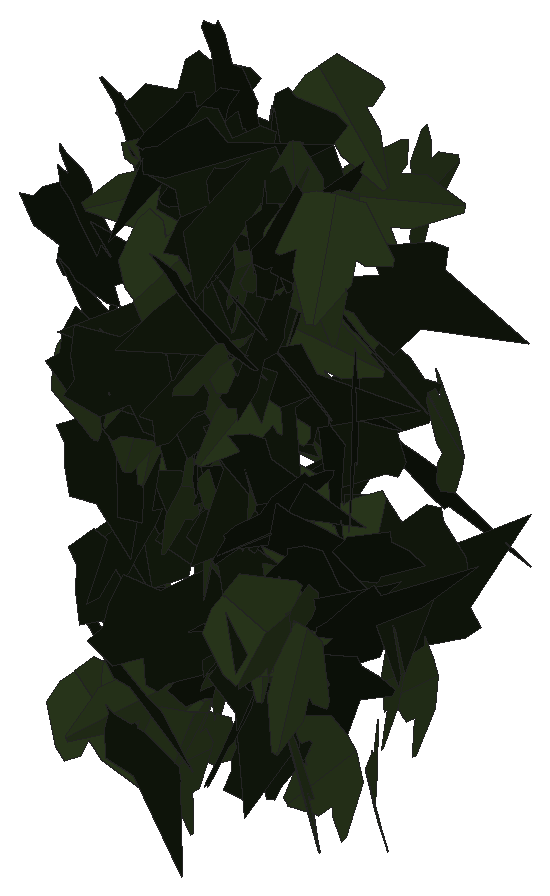
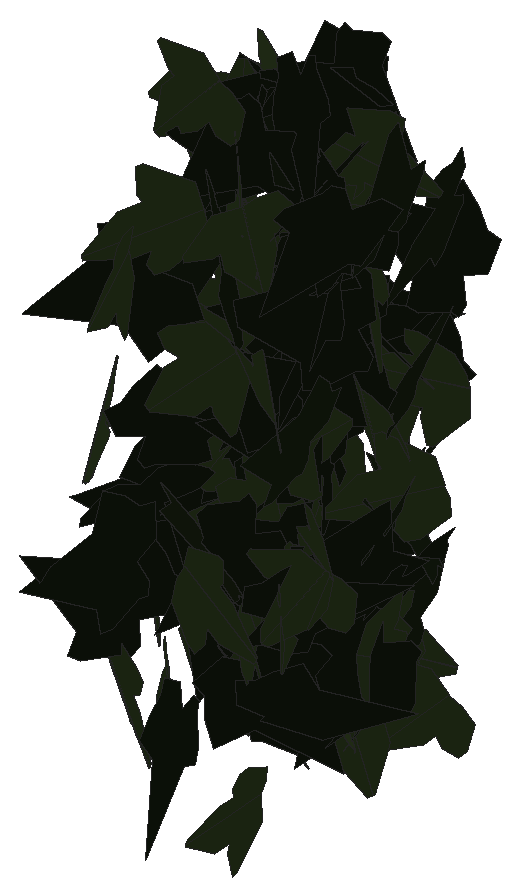
# SketchUp Ruby script. Lengths in inches.
U = 1.inch
M = Sketchup.active_model
def pt(a) = Geom::Point3d.new(a.map { |v| v * U })
def face(e, loops, mat)
  f = e.add_face(loops[0].map { |a| pt(a) })
  loops[1..].each { |l| e.add_face(l.map { |a| pt(a) }).erase! }
  f.material = f.back_material = mat if mat
  f
end
# faces: each face lists its corners as indices into pts; further lists are holes
def faces(e, pts, list, mat = nil) = list.each { |f| face(e, (f[0].is_a?(Array) ? f : [f]).map { |l| l.map { |i| pts[i] } }, mat) }
# xy, xz, yz: faces in a plane at the given z, y or x. An outline is a flat list of corners, or four numbers for a rectangle; further outlines are holes
def ring(l) = l.size == 4 ? [[l[0], l[1]], [l[2], l[1]], [l[2], l[3]], [l[0], l[3]]] : l.each_slice(2).to_a
def flat(e, list, mat, &to3) = list.each { |f| face(e, (f[0].is_a?(Array) ? f : [f]).map { |l| ring(l).map { |u, v| to3.(u, v) } }, mat) }
def xy(e, z, list, mat = nil) = flat(e, list, mat) { |x, y| [x, y, z] }
def xz(e, y, list, mat = nil) = flat(e, list, mat) { |x, z| [x, y, z] }
def yz(e, x, list, mat = nil) = flat(e, list, mat) { |y, z| [x, y, z] }
def lines(e, pts, list) = list.each { |a, b| e.add_line(pt(pts[a]), pt(pts[b])) }
# prism: a flat outline (further loops are holes) pulled along v
def prism(e, loops, v, mat = nil)
  f = face(e, loops, mat); d = Geom::Vector3d.new(v.map { |x| x * U })
  f.pushpull(f.normal.samedirection?(d) ? d.length : -d.length)
end
def box(e, o, s, mat = nil) = prism(e, [[o, [o[0] + s[0], o[1], o[2]], [o[0] + s[0], o[1] + s[1], o[2]], [o[0], o[1] + s[1], o[2]]]], [0, 0, s[2]], mat)
def at(x, y, z, deg = 0) = Geom::Transformation.translation(pt([x, y, z])) * Geom::Transformation.rotation(ORIGIN, Z_AXIS, deg.degrees)
def axes(o, x, y, z) = Geom::Transformation.new([*x, 0, *y, 0, *z, 0, *pt(o).to_a, 1])
def part(name) = M.definitions.add(name)
# library, detail: a bought-in or finely detailed component or shape, given as its bounding box
def library(name, o, s) = part(name).tap { |d| box(d.entities, o, s) }
def detail(e, o, s) = box(e.add_group.entities, o, s)
def put(e, d, t, mat = nil) = e.add_instance(d, t).tap { |i| i.material = mat if mat }
def group(e, t, mat = nil) = e.add_group.tap { |g| g.transformation = t; g.material = mat if mat }.entities
root = M.entities
M.materials.add("efeu1").color = [18, 25, 13]
M.materials.add("efeu2").color = [43, 57, 29]
c1 = part("ivyleaf_9")
p = [[1.54,2.16,1.25],[1.36,2.04,1.19],[-0.21,0.99,0.68],[-0.71,1.11,0.82],[-0.85,0.86,0.67],[-0.8,0.17,0.21],
  [-0.9,-0.01,0.1],[-0.67,-0.16,-0.02],[-0.08,-0.08,-0.05],[-0.03,-0.6,-0.4],[0.65,-0.88,-0.66],[0.83,-0.6,-0.49],
  [1.29,-0.42,-0.43],[1.8125,-0.07,-0.26],[1.21,0.44,0.15]]
faces(c1.entities,p,[[0,1,2,3,4,5,6,7,8,9,10,11,12,13,14]],"efeu1")
c2 = part("ivyleaf_10")
p = [[0,0.5,-0.03],[-0.0625,2.02,-0.43],[-0.19,2.01,-0.46],[-0.54,1.05,-0.29],[-0.52,0.625,-0.18],[-0.83,0.76,-0.28],
  [-1.16,0.64,-0.33],[-1.15,0.33,-0.24],[-0.77,-0.39,0.02],[-0.3,-0.51,0.16],[0.04,-0.48,0.23],[-0.02,2.01,-0.4375],
  [-0.06,2.01,-0.43],[0.04,-0.49,0.23],[0.67,-0.49,0.14],[1.38,0.36,-0.2],[1.375,0.51,-0.24],[0.81,0.65,-0.19],
  [0.62,0.59,-0.15],[0.6,1.09,-0.28],[0.5,1.23,-0.31]]
faces(c2.entities,p,[[0,1,2,3,4,5,6,7,8,9,10],[11,12,0,13,14,15,16,17,18,19,20]],"efeu2")
put(root,c1,axes([28.6875,223.91,213.04],[0.40877,-0.21276,-0.19401],[-0.17176,0.09021,-0.46083],[0.2311,0.44339,0.00067]))
put(root,c1,axes([28.94,224.4375,210.86],[0.14407,-0.45026,0.16281],[-0.02186,0.16366,0.47195],[-0.47829,-0.14311,0.02747]))
put(root,c2,axes([28.55,224.56,210.09],[0.11847,0.08591,0.47811],[0.33881,0.33804,-0.1447],[-0.3481,0.35826,0.02188]))
put(root,c2,axes([28.97,226.4375,211.65],[0.40883,-0.22984,0.17329],[-0.15126,0.08456,0.46901],[-0.2449,-0.43592,-0.00038]))
put(root,c1,axes([28.55,223.95,212.3],[0.14856,-0.10104,0.46661],[0.392,-0.25313,-0.17962],[0.27252,0.41919,0.004]))
put(root,c1,axes([28.66,226.22,211.32],[0.30316,-0.37641,0.12809],[0.08821,-0.09339,-0.48321],[0.3877,0.31558,0.00978]))
put(root,c1,axes([28.73,224.88,213.16],[0.3783,-0.19985,-0.25874],[0.22756,-0.12317,0.42784],[-0.23474,-0.44146,-0.00224]))
put(root,c2,axes([28.67,224.14,207.4375],[0.33561,0.08296,0.36123],[0.34168,0.11955,-0.34491],[-0.14359,0.47836,0.02355]))
put(root,c2,axes([28.94,224.81,208.15],[0.07535,-0.22845,0.43833],[0.17161,-0.40372,-0.23991],[0.46354,0.1866,0.01757]))
put(root,c1,axes([28.87,225.29,213.42],[-0.00267,-0.238,-0.43971],[0.03683,0.43843,-0.23753],[0.49863,-0.03366,0.01519]))
put(root,c2,axes([28.78,225.85,209.67],[-0.0462,0.07315,-0.49246],[0.30942,-0.38324,-0.08596],[-0.39003,-0.3127,-0.00985]))
put(root,c1,axes([29.32,225.95,208.99],[-0.21599,-0.12914,0.43205],[-0.37674,-0.21159,-0.25159],[0.24781,-0.43423,-0.0059]))
put(root,c1,axes([28.89,224.73,209.64],[-0.05666,-0.22028,0.44527],[0.06937,-0.44727,-0.21245],[0.49191,0.03771,0.08125]))
put(root,c1,axes([28.94,224.74,208.25],[0.44801,0.21995,-0.03005],[-0.03031,-0.00644,-0.49904],[-0.21992,0.44898,0.00756]))
put(root,c2,axes([28.69,224,210.99],[-0.07061,-0.0021,-0.49498],[0.48693,-0.09017,-0.06907],[-0.08898,-0.4918,0.01478]))
put(root,c1,axes([28.83,224.09,210.17],[0.25674,-0.42821,-0.0269],[-0.01511,0.0223,-0.49927],[0.42878,0.25718,-0.00149]))
put(root,c1,axes([28.89,224.33,208.97],[0.17941,-0.4226,-0.19804],[-0.06084,0.18918,-0.45881],[0.46272,0.18873,0.01646]))
put(root,c1,axes([29.44,225.82,207.77],[-0.26268,-0.03608,0.42391],[-0.41881,-0.06569,-0.26511],[0.07482,-0.49435,0.00429]))
put(root,c2,axes([28.82,225.89,209.52],[0.36416,0.17833,0.29255],[0.25167,0.15047,-0.40499],[-0.23248,0.44222,0.01983]))
put(root,c1,axes([29.33,224.9,209.03],[-0.41509,-0.26704,0.07993],[0.06882,0.04076,0.49356],[-0.27012,0.42074,0.00292]))
put(root,c1,axes([29.29,223.82,209.22],[-0.34413,0.32724,-0.15648],[-0.12117,0.0996,0.47476],[0.34189,0.36468,0.01075]))
put(root,c2,axes([29.15,224.22,207.93],[0.04653,0.30441,0.39392],[0.07018,0.38767,-0.30787],[-0.49286,0.08394,-0.00665]))
put(root,c2,axes([29.1875,224.55,210.8],[0.45106,-0.20553,0.06559],[0.06059,-0.0252,-0.49567],[0.20706,0.45511,0.00217]))
put(root,c1,axes([29.02,224.04,208.23],[0.37916,-0.32449,0.03065],[0.02319,-0.02004,-0.49906],[0.32511,0.37987,-0.00015]))
put(root,c2,axes([29.51,224.23,207.82],[-0.05387,-0.17407,0.46561],[-0.16039,-0.43721,-0.18201],[0.4705,-0.16897,-0.00874]))
put(root,c2,axes([29.25,225.58,210.72],[-0.00569,-0.05343,0.4971],[0.18139,-0.46349,-0.04774],[0.4659,0.17979,0.02466]))
put(root,c1,axes([29.05,223.89,210.89],[-0.10825,0.03471,0.48691],[0.43525,-0.21892,0.11237],[0.22099,0.44818,0.01718]))
put(root,c2,axes([29.41,225.48,209.28],[0.08997,-0.40958,-0.2723],[-0.02562,0.27254,-0.41841],[0.49117,0.08924,0.02805]))
put(root,c2,axes([29.47,224.28,212.13],[0.30868,-0.25758,-0.29727],[-0.16144,0.26162,-0.39433],[0.35868,0.33943,0.07834]))
put(root,c2,axes([29.5,224.03,211.05],[-0.38838,-0.28696,0.12967],[-0.10056,-0.08209,-0.48285],[0.29841,-0.40114,0.00605]))
put(root,c2,axes([29.74,226.64,209.48],[-0.1779,0.03813,0.46572],[-0.46728,-0.01242,-0.17747],[-0.00196,-0.49839,0.04005]))
put(root,c1,axes([29.63,225.82,208.24],[0.03233,0.22646,-0.4446],[-0.06196,-0.44026,-0.22875],[-0.49509,0.06988,-0.00041]))
put(root,c2,axes([29.6,224.46,207.27],[-0.28853,-0.38483,0.13659],[-0.07791,-0.1123,-0.48096],[0.40085,-0.29883,0.00484]))
put(root,c1,axes([29.62,224.64,209.93],[-0.00253,-0.06778,0.49538],[0.02287,0.49485,0.06782],[-0.49947,0.02301,0.0006]))
put(root,c2,axes([29.46,226.12,206.88],[0.05637,-0.01042,-0.4967],[0.09809,0.49028,0.00084],[0.48703,-0.09753,0.05732]))
put(root,c1,axes([29.82,224.6,211.49],[-0.2655,-0.05561,0.42002],[-0.39578,-0.14438,-0.26929],[0.15123,-0.47546,0.03265]))
put(root,c2,axes([29.84,224.08,213.33],[0.21481,0.03242,-0.45034],[-0.44683,-0.05629,-0.21719],[-0.06478,0.49576,0.00478]))
put(root,c1,axes([29.34,224.15,207.3],[0.19968,-0.45082,0.083],[0.03004,-0.07747,-0.49305],[0.45741,0.20189,-0.00386]))
put(root,c1,axes([30,224.03,211.42],[-0.41401,0.1922,0.2041],[-0.18692,0.08206,-0.45643],[-0.20895,-0.45423,0.0039]))
put(root,c1,axes([29.5,223.78,211.06],[-0.25682,-0.06376,0.42424],[0.42889,-0.02657,0.25564],[-0.01006,0.49521,0.06834]))
put(root,c1,axes([29.29,224.72,211.73],[0.2633,-0.00274,0.42505],[0.41926,0.08394,-0.25918],[-0.06993,0.4929,0.0465]))
put(root,c2,axes([29.74,224.28,210.02],[-0.00079,-0.27761,-0.41585],[-0.00374,0.41584,-0.2776],[0.49999,0.00267,-0.00274]))
put(root,c1,axes([29.5,224.58,210.52],[-0.09786,-0.05019,0.48775],[0.45227,0.18288,0.10956],[-0.1894,0.46264,0.00961]))
put(root,c2,axes([29.74,225.67,208.66],[0.09486,-0.48546,0.07298],[0.01243,-0.07194,-0.49464],[0.49076,0.09566,-0.00158]))
put(root,c1,axes([29.91,224.75,214.32],[0.24472,-0.00269,-0.43601],[-0.43568,-0.02129,-0.2444],[-0.01725,0.49954,-0.01277]))
put(root,c1,axes([29.8,226.81,208.08],[0.35829,-0.03495,-0.347],[-0.34354,0.05031,-0.35979],[0.06006,0.49623,0.01204]))
put(root,c1,axes([29.78,224.66,212.01],[0.39745,0.01618,-0.30294],[-0.30329,0.00961,-0.3974],[-0.00703,0.49965,0.01745]))
put(root,c1,axes([29.41,224.85,213.02],[0.09089,0.00062,-0.49167],[0.48585,0.07658,0.08991],[0.07542,-0.4941,0.01332]))
put(root,c2,axes([29.64,224.42,206.95],[0.14649,-0.26393,-0.3986],[0.25004,-0.31302,0.29916],[-0.40745,-0.28698,0.04028]))
put(root,c1,axes([29.99,224.07,214.15],[-0.16598,0.25068,-0.39951],[0.16631,-0.36521,-0.29826],[-0.44135,-0.2319,0.03785]))
put(root,c2,axes([29.93,224.82,208.23],[0.15791,-0.47423,0.01321],[0.00575,-0.01201,-0.49982],[0.47438,0.158,0.00166]))
put(root,c2,axes([29.8,223.67,212.47],[0.10819,0.14501,-0.46612],[0.19938,0.42267,0.17777],[0.44558,-0.22434,0.03363]))
put(root,c1,axes([29.77,224.625,213.1],[0.10667,-0.48539,0.05497],[0.02093,-0.05167,-0.49688],[0.48804,0.1083,0.0093]))
put(root,c1,axes([29.8,223.64,208.53],[-0.08086,-0.04364,0.49149],[0.44785,0.20256,0.09166],[-0.20711,0.45504,0.00633]))
put(root,c1,axes([29.61,224.05,212.23],[0.3623,-0.20993,0.27326],[0.22741,-0.15222,-0.41846],[0.25889,0.4275,-0.01482]))
put(root,c1,axes([30.01,224.9375,209.36],[-0.28796,-0.4058,-0.04906],[0.03187,0.03754,-0.49757],[0.40751,-0.28969,0.00425]))
put(root,c1,axes([29.78,224.46,210.13],[0.09161,0.07138,0.48633],[0.42822,0.23128,-0.11461],[-0.24132,0.43751,-0.01876]))
put(root,c1,axes([30.29,224.27,213.32],[-0.24951,0.43218,-0.03108],[0.01446,-0.02754,-0.49903],[-0.43305,-0.24993,0.00124]))
put(root,c1,axes([30.2,224.5625,212.04],[-0.19858,-0.23718,0.39283],[-0.25782,-0.29641,-0.3093],[0.37959,-0.3254,-0.00458]))
put(root,c1,axes([29.84,225.39,208.2],[0.2917,-0.39803,-0.08052],[-0.04764,0.06492,-0.49347],[0.40329,0.29556,-0.00005]))
put(root,c1,axes([29.9375,224.5,211.25],[0.04816,-0.19123,-0.45947],[-0.05156,0.45722,-0.19569],[0.495,0.06623,0.02432]))
put(root,c1,axes([30.08,225.32,209.34],[-0.04537,0.08926,-0.48987],[-0.17407,0.45802,0.09958],[0.46652,0.17958,-0.01049]))
put(root,c1,axes([29.82,224.26,208.08],[0.20032,0.39611,-0.23016],[0.06641,0.22344,0.44234],[0.45328,-0.20779,0.03691]))
put(root,c2,axes([30.07,225.42,212.98],[0.24779,0.41999,-0.11048],[-0.06825,-0.08796,-0.48745],[-0.42889,0.25665,0.01374]))
put(root,c1,axes([30.28,225.78,209.38],[-0.37089,0.3283,-0.06828],[-0.05185,0.04444,0.49531],[0.33129,0.37449,0.00108]))
put(root,c2,axes([29.97,224.47,209.85],[0.09486,-0.22614,0.43573],[0.3067,-0.31922,-0.23245],[0.38333,0.31138,0.07815]))
put(root,c2,axes([30.34,224.32,211.59],[-0.11753,-0.48591,0.00907],[-0.00019,-0.00929,-0.49991],[0.48599,-0.11751,0.00199]))
put(root,c1,axes([30.3,224.73,206.97],[-0.35476,0.34495,0.0718],[0.04566,-0.05602,0.49475],[0.34937,0.35759,0.00825]))
put(root,c2,axes([30.37,224.29,212.59],[0.05732,-0.17254,-0.46577],[-0.02628,0.46716,-0.17628],[0.49601,0.04469,0.04448]))
put(root,c1,axes([30.51,223.97,207.67],[-0.02477,0.31413,0.38821],[-0.02534,0.3874,-0.31509],[-0.49874,-0.03528,-0.00327]))
put(root,c1,axes([30.02,223.84,213.58],[0.21223,0.02266,0.45216],[0.42721,0.15525,-0.2083],[-0.14984,0.47475,0.04654]))
put(root,c1,axes([30.25,224.58,212.4],[-0.16856,-0.41738,-0.21767],[0.08876,0.19887,-0.45008],[0.46229,-0.19037,0.00705]))
put(root,c1,axes([30.35,224.16,213.9],[-0.32847,-0.34431,-0.15349],[0.10632,0.11071,-0.47586],[0.36167,-0.34525,0.00049]))
put(root,c1,axes([30.01,225,211.02],[0.42105,-0.03551,0.26731],[0.26844,0.00818,-0.42175],[0.02557,0.49867,0.02595]))
put(root,c2,axes([30.34,224.625,209.34],[-0.14243,-0.47889,0.01953],[0.00567,0.01869,0.49962],[-0.47925,0.14254,0.0001]))
put(root,c1,axes([30.2,224.56,211.22],[-0.19438,-0.14987,-0.43561],[0.34224,0.26951,-0.24544],[0.30837,-0.39358,-0.00219]))
put(root,c1,axes([30.28,224.66,209.49],[-0.01735,-0.47464,0.15627],[0.00776,-0.1566,-0.47478],[0.49964,-0.01405,0.0128]))
put(root,c2,axes([30.2,225.74,211.46],[-0.36429,0.0383,-0.34033],[0.33866,-0.03372,-0.3663],[-0.05101,-0.49739,-0.00137]))
put(root,c1,axes([30.4375,224.77,210.21],[-0.16029,-0.36462,0.30226],[-0.10713,-0.28292,-0.39809],[0.46134,-0.19238,0.01258]))
put(root,c2,axes([30.18,224.53,210.08],[-0.15156,0.09079,0.46775],[0.40528,-0.23354,0.17665],[0.25055,0.43268,-0.0028]))
put(root,c1,axes([30.36,225.18,211.77],[-0.08678,0.3659,0.32952],[-0.00467,-0.3352,0.37097],[0.49239,0.06131,0.0616]))
put(root,c1,axes([30.37,223.91,213.36],[0.01197,0.04606,-0.49773],[-0.08942,0.49004,0.04319],[0.49179,0.08798,0.01997]))
put(root,c2,axes([30.56,224.51,211.3125],[0.19895,0.28324,-0.36083],[-0.21311,-0.29121,-0.34609],[-0.40621,0.2915,0.00485]))
put(root,c2,axes([30.77,224.71,213],[-0.06373,0.03355,0.49479],[-0.4038,0.28609,-0.07141],[-0.2879,-0.40869,-0.00938]))
put(root,c1,axes([30.24,224.95,213.71],[-0.09489,-0.1152,-0.4772],[0.32381,0.35063,-0.14903],[0.36898,-0.33733,0.00806]))
put(root,c1,axes([30.23,224.41,212.13],[0.40285,-0.2763,0.10665],[0.08954,-0.05802,-0.48848],[0.28231,0.41267,0.00273]))
put(root,c1,axes([30.4,224.72,207.84],[0.00704,-0.43984,0.23768],[0.00015,-0.23771,-0.43988],[0.49995,0.00626,-0.00322]))
put(root,c1,axes([30.88,224,211.9],[-0.31275,0.12802,-0.36851],[-0.34061,0.14066,0.33793],[0.19019,0.46241,-0.00077]))
put(root,c2,axes([30.47,224.42,209.07],[0.43995,-0.13416,0.19608],[0.19008,-0.04879,-0.45988],[0.14253,0.47919,0.00807]))
put(root,c1,axes([30.31,224.22,210.42],[0.1757,0.12302,-0.45166],[0.37229,0.25573,0.21448],[0.28378,-0.41166,-0.00174]))
put(root,c1,axes([31,225.76,210.39],[-0.08818,-0.01067,0.49205],[-0.46214,-0.17013,-0.08651],[0.16927,-0.47004,0.02015]))
put(root,c2,axes([30.86,226.35,212.58],[0.03998,-0.09045,-0.49012],[-0.04413,0.48912,-0.09386],[0.49644,0.05076,0.03112]))
put(root,c1,axes([30.91,223.96,210.25],[0.08053,0.48341,0.09913],[0.01659,0.09773,-0.49007],[-0.49319,0.08222,-0.0003]))
put(root,c2,axes([30.84,224.58,213.05],[-0.35705,-0.34564,-0.05522],[-0.03967,-0.03841,0.49694],[-0.34776,0.35925,0.00001]))
put(root,c1,axes([30.94,224.14,212.83],[-0.03579,-0.27273,0.41754],[0.07851,0.41031,0.27474],[-0.4925,0.08523,0.01345]))
put(root,c2,axes([30.8,224.58,207.46],[-0.30834,0.38043,-0.101],[0.06319,-0.07879,-0.48969],[-0.3885,-0.31475,0.00051]))
put(root,c2,axes([31,224.83,209.54],[0.34157,0.28527,0.22793],[-0.18453,-0.13446,0.44483],[0.31509,-0.388,0.01342]))
put(root,c2,axes([30.73,224.64,209],[0.19497,0.39647,0.23408],[0.08661,0.21808,-0.44152],[-0.4522,0.21271,0.01636]))
put(root,c2,axes([30.49,225.01,211.5625],[-0.00872,0.00218,0.49992],[0.49097,0.09424,0.00815],[-0.09418,0.49103,-0.00378]))
put(root,c1,axes([30.55,226.63,209.48],[0.43018,-0.17661,0.18371],[0.17304,-0.06216,-0.46497],[0.18708,0.46362,0.00764]))
put(root,c1,axes([30.6,224.59,208.59],[0.32608,0.3512,-0.14259],[0.0974,0.10413,0.47924],[0.36631,-0.34031,-0.00051]))
put(root,c1,axes([30.54,224.46,211.17],[0.284,0.02139,0.41096],[0.41113,0.00688,-0.28448],[-0.01782,0.4995,-0.01368]))
put(root,c1,axes([30.71,224.3,209.91],[0.48923,0.07351,0.07248],[0.07192,0.00913,-0.49472],[-0.07405,0.49448,-0.00164]))
put(root,c2,axes([30.79,225.6,212.84],[0.07178,0.07882,0.4885],[0.1643,0.46181,-0.09866],[-0.46675,0.17469,0.0404]))
put(root,c2,axes([31.19,226,207.7],[0.2195,-0.23302,-0.38408],[-0.26406,0.27891,-0.32012],[0.36345,0.34338,-0.00062]))
put(root,c1,axes([31.01,224.47,208.4],[0.33504,0.33909,-0.15087],[-0.11616,-0.09723,-0.4765],[-0.35249,0.35435,0.01363]))
put(root,c2,axes([30.72,225.18,214.14],[0.34945,0.03624,0.35577],[0.34552,0.09405,-0.34896],[-0.09222,0.48974,0.04069]))
put(root,c2,axes([31.25,224.64,207.4375],[0.34113,-0.17149,-0.32284],[-0.28484,0.15207,-0.38176],[0.22912,0.44437,0.00606]))
put(root,c2,axes([30.75,223.85,209.16],[0.23807,0.11772,0.42363],[0.36023,0.22399,-0.26469],[-0.2521,0.43124,0.02184]))
put(root,c1,axes([31.03,224.01,212.97],[0.07577,0.06217,0.4903],[0.24813,0.42419,-0.09214],[-0.42742,0.25728,0.03343]))
put(root,c2,axes([31.16,224.01,209.13],[-0.00885,-0.46826,-0.17509],[-0.00702,0.17521,-0.46824],[0.49987,-0.00583,-0.00968]))
put(root,c2,axes([31.13,223.62,213.17],[0.2199,-0.27535,0.35472],[-0.12005,0.34454,0.34188],[-0.4327,-0.23552,0.08542]))
put(root,c2,axes([31.36,224.25,212.9],[0.32276,-0.09221,-0.37057],[-0.30874,0.22253,-0.32428],[0.22473,0.43815,0.08671]))
put(root,c1,axes([31.24,224.58,209.66],[0.22964,0.41977,-0.14511],[-0.07385,-0.12499,-0.47846],[-0.43796,0.24118,0.00459]))
put(root,c1,axes([31.01,224.83,210.28],[-0.04225,0.08341,0.49118],[0.11165,-0.47882,0.09091],[0.48554,0.11736,0.02184]))
put(root,c2,axes([31.54,224.88,207.03],[-0.08445,0.06726,0.4882],[-0.41225,0.26177,-0.10738],[-0.27003,-0.42066,0.01124]))
put(root,c1,axes([31.0625,225.9375,208.38],[-0.03099,-0.02906,0.49819],[0.45463,0.20419,0.04019],[-0.20579,0.45548,0.01377]))
put(root,c1,axes([31,224.76,212.27],[0.44003,-0.22226,0.0835],[0.07505,-0.03662,-0.49298],[0.22526,0.44638,0.00114]))
put(root,c1,axes([31.05,225.6,212.1],[0.05234,0.06792,-0.49259],[0.27022,0.41191,0.0855],[0.41742,-0.27517,0.00641]))
put(root,c2,axes([31.35,223.9,208.95],[0.47706,-0.14865,0.01782],[0.01715,-0.00487,-0.49968],[0.14873,0.47737,0.00045]))
put(root,c2,axes([31.38,226.18,210.17],[-0.28655,0.32553,0.24883],[0.15299,-0.19668,0.43349],[0.38011,0.32457,0.01311]))
put(root,c1,axes([31.32,225.5,209.56],[-0.1045,-0.47857,-0.10027],[0.02681,0.09677,-0.48981],[0.48822,-0.10774,0.00543]))
put(root,c1,axes([31.3,224.85,211.34],[-0.05827,-0.00207,-0.49659],[0.46518,-0.17523,-0.05385],[-0.17381,-0.46829,0.02235]))
put(root,c2,axes([31.71,224.91,208.42],[0.16782,-0.24019,-0.40515],[-0.20818,0.34798,-0.29253],[0.42249,0.26687,0.01679]))
put(root,c2,axes([31.48,224.22,213.46],[0.47187,0.16362,-0.02379],[-0.02238,-0.00808,-0.49943],[-0.16382,0.4724,-0.0003]))
put(root,c1,axes([31.375,224.51,208.87],[0.02136,0.40337,-0.29467],[0.00211,0.29487,0.40379],[0.49954,-0.01849,0.01089]))
